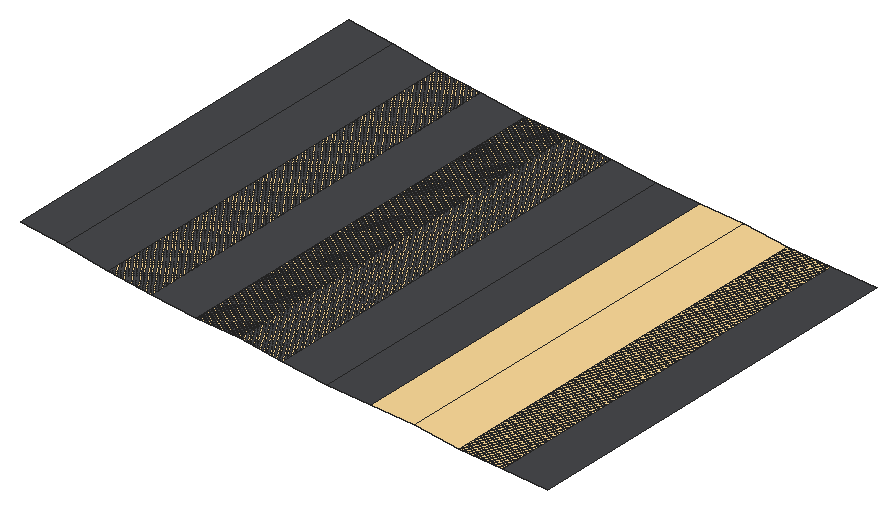
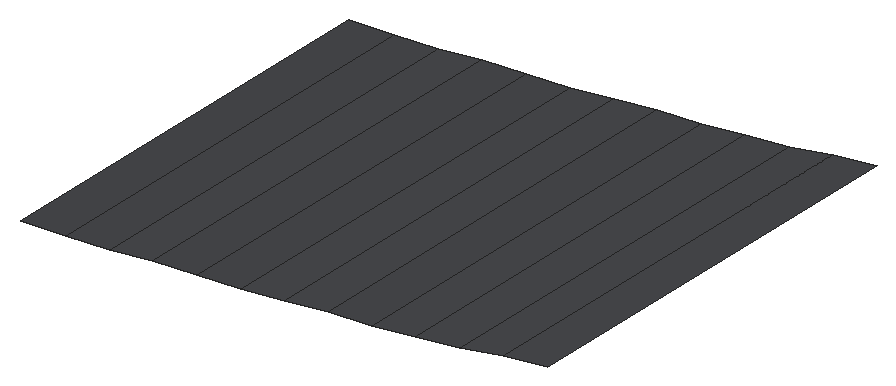
# SketchUp Ruby script. Lengths in inches.
U = 1.inch
M = Sketchup.active_model
def pt(a) = Geom::Point3d.new(a.map { |v| v * U })
def face(e, loops, mat)
  f = e.add_face(loops[0].map { |a| pt(a) })
  loops[1..].each { |l| e.add_face(l.map { |a| pt(a) }).erase! }
  f.material = f.back_material = mat if mat
  f
end
# faces: each face lists its corners as indices into pts; further lists are holes
def faces(e, pts, list, mat = nil) = list.each { |f| face(e, (f[0].is_a?(Array) ? f : [f]).map { |l| l.map { |i| pts[i] } }, mat) }
# xy, xz, yz: faces in a plane at the given z, y or x. An outline is a flat list of corners, or four numbers for a rectangle; further outlines are holes
def ring(l) = l.size == 4 ? [[l[0], l[1]], [l[2], l[1]], [l[2], l[3]], [l[0], l[3]]] : l.each_slice(2).to_a
def flat(e, list, mat, &to3) = list.each { |f| face(e, (f[0].is_a?(Array) ? f : [f]).map { |l| ring(l).map { |u, v| to3.(u, v) } }, mat) }
def xy(e, z, list, mat = nil) = flat(e, list, mat) { |x, y| [x, y, z] }
def xz(e, y, list, mat = nil) = flat(e, list, mat) { |x, z| [x, y, z] }
def yz(e, x, list, mat = nil) = flat(e, list, mat) { |y, z| [x, y, z] }
def lines(e, pts, list) = list.each { |a, b| e.add_line(pt(pts[a]), pt(pts[b])) }
# prism: a flat outline (further loops are holes) pulled along v
def prism(e, loops, v, mat = nil)
  f = face(e, loops, mat); d = Geom::Vector3d.new(v.map { |x| x * U })
  f.pushpull(f.normal.samedirection?(d) ? d.length : -d.length)
end
def box(e, o, s, mat = nil) = prism(e, [[o, [o[0] + s[0], o[1], o[2]], [o[0] + s[0], o[1] + s[1], o[2]], [o[0], o[1] + s[1], o[2]]]], [0, 0, s[2]], mat)
def at(x, y, z, deg = 0) = Geom::Transformation.translation(pt([x, y, z])) * Geom::Transformation.rotation(ORIGIN, Z_AXIS, deg.degrees)
def axes(o, x, y, z) = Geom::Transformation.new([*x, 0, *y, 0, *z, 0, *pt(o).to_a, 1])
def part(name) = M.definitions.add(name)
# library, detail: a bought-in or finely detailed component or shape, given as its bounding box
def library(name, o, s) = part(name).tap { |d| box(d.entities, o, s) }
def detail(e, o, s) = box(e.add_group.entities, o, s)
def put(e, d, t, mat = nil) = e.add_instance(d, t).tap { |i| i.material = mat if mat }
def group(e, t, mat = nil) = e.add_group.tap { |g| g.transformation = t; g.material = mat if mat }.entities
root = M.entities
M.materials.add("1432 AP 8245 TAR ROAD").color = [71, 72, 75]
M.materials.add("Outer Light").color = [251, 217, 152]
p = [[277.39,95.37,171.36],[277.55,95.37,171.34],[277.55,96.87,171.34],[277.39,96.87,171.36],[277.39,96.87,171.36],[277.55,96.87,171.34],
  [277.55,95.37,171.34],[277.39,95.37,171.36],[277.71,95.37,171.33],[277.71,96.87,171.33],[277.71,96.87,171.33],[277.71,95.37,171.33],
  [277.875,95.37,171.32],[277.875,96.87,171.32],[276.43,95.37,171.45],[276.59,95.37,171.43],[276.59,96.87,171.43],[276.43,96.87,171.45],
  [276.43,96.87,171.45],[276.59,96.87,171.43],[276.59,95.37,171.43],[276.43,95.37,171.45],[276.75,95.37,171.42],[276.75,96.87,171.42],
  [276.75,96.87,171.42],[276.75,95.37,171.42],[276.91,95.37,171.4],[276.91,96.87,171.4],[276.91,96.87,171.4],[276.91,95.37,171.4],
  [277.07,95.37,171.38],[277.07,96.87,171.38],[277.07,96.87,171.38],[277.07,95.37,171.38],[277.23,95.37,171.37],[277.23,96.87,171.37],
  [277.23,96.87,171.37],[277.23,95.37,171.37],[275.95,95.37,171.52],[276.11,95.37,171.5],[276.11,96.87,171.5],[275.95,96.87,171.52],
  [275.95,96.87,171.52],[276.11,96.87,171.5],[276.11,95.37,171.5],[275.95,95.37,171.52],[276.27,95.37,171.47],[276.27,96.87,171.47],
  [276.27,96.87,171.47],[276.27,95.37,171.47]]
faces(root,p,[[0,1,2,3],[1,8,9,2],[8,12,13,9],[14,15,16,17],[15,22,23,16],[22,26,27,23],[26,30,31,27],[30,34,35,31],
  [34,0,3,35],[38,39,40,41],[39,46,47,40],[46,14,17,47]],"1432 AP 8245 TAR ROAD")
faces(root,p,[[4,5,6,7],[5,10,11,6],[18,19,20,21],[19,24,25,20],[24,28,29,25],[28,32,33,29],[32,36,37,33],[36,4,7,37],
  [42,43,44,45],[43,48,49,44],[48,18,21,49]],"Outer Light")
